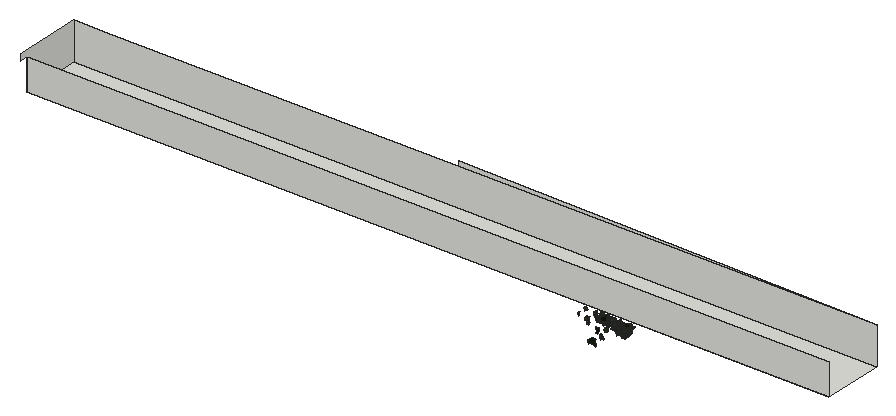
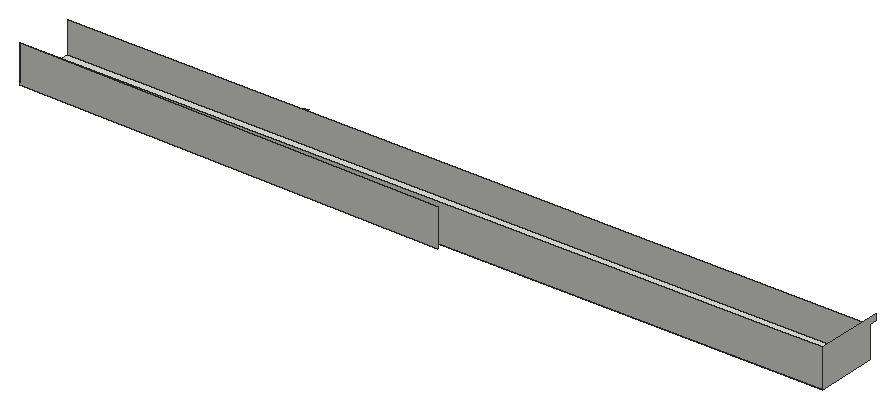
# SketchUp Ruby script. Lengths in inches.
U = 1.inch
M = Sketchup.active_model
def pt(a) = Geom::Point3d.new(a.map { |v| v * U })
def face(e, loops, mat)
  f = e.add_face(loops[0].map { |a| pt(a) })
  loops[1..].each { |l| e.add_face(l.map { |a| pt(a) }).erase! }
  f.material = f.back_material = mat if mat
  f
end
# faces: each face lists its corners as indices into pts; further lists are holes
def faces(e, pts, list, mat = nil) = list.each { |f| face(e, (f[0].is_a?(Array) ? f : [f]).map { |l| l.map { |i| pts[i] } }, mat) }
# xy, xz, yz: faces in a plane at the given z, y or x. An outline is a flat list of corners, or four numbers for a rectangle; further outlines are holes
def ring(l) = l.size == 4 ? [[l[0], l[1]], [l[2], l[1]], [l[2], l[3]], [l[0], l[3]]] : l.each_slice(2).to_a
def flat(e, list, mat, &to3) = list.each { |f| face(e, (f[0].is_a?(Array) ? f : [f]).map { |l| ring(l).map { |u, v| to3.(u, v) } }, mat) }
def xy(e, z, list, mat = nil) = flat(e, list, mat) { |x, y| [x, y, z] }
def xz(e, y, list, mat = nil) = flat(e, list, mat) { |x, z| [x, y, z] }
def yz(e, x, list, mat = nil) = flat(e, list, mat) { |y, z| [x, y, z] }
def lines(e, pts, list) = list.each { |a, b| e.add_line(pt(pts[a]), pt(pts[b])) }
# prism: a flat outline (further loops are holes) pulled along v
def prism(e, loops, v, mat = nil)
  f = face(e, loops, mat); d = Geom::Vector3d.new(v.map { |x| x * U })
  f.pushpull(f.normal.samedirection?(d) ? d.length : -d.length)
end
def box(e, o, s, mat = nil) = prism(e, [[o, [o[0] + s[0], o[1], o[2]], [o[0] + s[0], o[1] + s[1], o[2]], [o[0], o[1] + s[1], o[2]]]], [0, 0, s[2]], mat)
def at(x, y, z, deg = 0) = Geom::Transformation.translation(pt([x, y, z])) * Geom::Transformation.rotation(ORIGIN, Z_AXIS, deg.degrees)
def axes(o, x, y, z) = Geom::Transformation.new([*x, 0, *y, 0, *z, 0, *pt(o).to_a, 1])
def part(name) = M.definitions.add(name)
# library, detail: a bought-in or finely detailed component or shape, given as its bounding box
def library(name, o, s) = part(name).tap { |d| box(d.entities, o, s) }
def detail(e, o, s) = box(e.add_group.entities, o, s)
def put(e, d, t, mat = nil) = e.add_instance(d, t).tap { |i| i.material = mat if mat }
def group(e, t, mat = nil) = e.add_group.tap { |g| g.transformation = t; g.material = mat if mat }.entities
root = M.entities
M.materials.add("efeu1").color = [18, 25, 13]
M.materials.add("efeu2").color = [43, 57, 29]
c1 = part("ivyleaf_10")
p = [[0,0.5,-0.03],[-0.0625,2.02,-0.43],[-0.19,2.01,-0.46],[-0.54,1.05,-0.29],[-0.52,0.625,-0.18],[-0.83,0.76,-0.28],
  [-1.16,0.64,-0.33],[-1.15,0.33,-0.24],[-0.77,-0.39,0.02],[-0.3,-0.51,0.16],[0.04,-0.48,0.23],[-0.02,2.01,-0.4375],
  [-0.06,2.01,-0.43],[0.04,-0.49,0.23],[0.67,-0.49,0.14],[1.38,0.36,-0.2],[1.375,0.51,-0.24],[0.81,0.65,-0.19],
  [0.62,0.59,-0.15],[0.6,1.09,-0.28],[0.5,1.23,-0.31]]
faces(c1.entities,p,[[0,1,2,3,4,5,6,7,8,9,10],[11,12,0,13,14,15,16,17,18,19,20]],"efeu2")
c2 = part("ivyleaf_9")
p = [[1.54,2.16,1.25],[1.36,2.04,1.19],[-0.21,0.99,0.68],[-0.71,1.11,0.82],[-0.85,0.86,0.67],[-0.8,0.17,0.21],
  [-0.9,-0.01,0.1],[-0.67,-0.16,-0.02],[-0.08,-0.08,-0.05],[-0.03,-0.6,-0.4],[0.65,-0.88,-0.66],[0.83,-0.6,-0.49],
  [1.29,-0.42,-0.43],[1.8125,-0.07,-0.26],[1.21,0.44,0.15]]
faces(c2.entities,p,[[0,1,2,3,4,5,6,7,8,9,10,11,12,13,14]],"efeu1")
xy(root,154.12,[[244.11,139.97,243.67,166.9375,600,172.6875,600.44,145.72]])
xz(root,172.6875,[[412.26,154.12,600,171.1]])
p = [[243.67,166.9375,171.1],[243.67,166.9375,154.12],[244.11,139.97,154.12],[244.11,139.97,168.16],[244.16,136.53,168.16],[244.16,136.53,171.1],
  [600.44,145.72,154.12],[600.44,145.72,168.16],[260.85,167.21,171.1],[600,172.6875,171.1],[600,172.6875,154.12]]
faces(root,p,[[0,1,2,3,4,5],[6,7,3,2],[8,9,10,1,0]])
put(root,c1,axes([494.1875,137.87,154.14],[0.47272,-0.38948,0.22707],[0.17708,-0.14216,-0.6125],[0.41461,0.50479,0.0027]))
put(root,c1,axes([496.87,138.41,156.75],[0.62684,-0.04431,-0.10252],[-0.10228,0.00702,-0.6284],[0.04486,0.63513,-0.0002]))
put(root,c1,axes([499.58,135.4,155.04],[0.33148,0.54304,0.37357],[0.1941,0.31919,-0.63621],[-0.6299,0.38412,0.00054]))
put(root,c1,axes([499.91,135.4,153.21],[0.19119,-0.08958,-0.71251],[0.63493,-0.3234,0.21103],[-0.33551,-0.66305,-0.00667]))
put(root,c1,axes([501.62,137.51,156.94],[-0.27922,-0.41477,-0.49379],[0.27947,0.4071,-0.49998],[0.58117,-0.39503,0.00319]))
put(root,c1,axes([502.09,137.56,154.76],[-0.31674,0.08852,0.62038],[0.60112,-0.15355,0.32881],[0.17712,0.67943,-0.00652]))
put(root,c1,axes([503.05,137.92,153.99],[-0.42973,-0.39488,-0.26374],[0.17751,0.19634,-0.58319],[0.44044,-0.46442,-0.0223]))
put(root,c1,axes([503.26,139.19,156.5],[0.20128,-0.51218,-0.35191],[-0.0623,0.35141,-0.5471],[0.6183,0.20214,0.05944]))
put(root,c1,axes([503.68,138.32,157],[-0.08296,-0.35065,-0.52599],[0.15228,0.50379,-0.35987],[0.61354,-0.17245,0.0182]))
put(root,c1,axes([503.71,138.3,154.38],[-0.2872,0.56478,-0.06141],[0.02675,-0.05529,-0.63361],[-0.56748,-0.28844,0.00121]))
put(root,c1,axes([503.36,136.47,155.96],[-0.12078,0.02245,-0.72965],[0.7174,-0.13318,-0.12285],[-0.13505,-0.72749,-0.00003]))
put(root,c1,axes([503.96,138.3,156.6],[0.02561,-0.2422,-0.61075],[0.13944,0.5993,-0.23181],[0.64206,-0.1205,0.07471]))
put(root,c1,axes([504.64,138.72,153.97],[0.20829,-0.57579,0.19315],[0.0493,-0.18749,-0.61208],[0.60532,0.2134,-0.01661]))
put(root,c1,axes([504.8,138.11,155.21],[0.04315,0.54456,0.35881],[0.03766,0.35691,-0.54621],[-0.65105,0.05674,-0.00781]))
put(root,c1,axes([504.82,138.46,154.46],[0.01472,-0.12796,0.64505],[0.58115,-0.29945,-0.07267],[0.30778,0.57152,0.10635]))
put(root,c1,axes([505.3,138.68,155.97],[0.04591,-0.0821,0.63986],[0.31247,-0.55838,-0.09406],[0.56438,0.31582,0.00003]))
put(root,c1,axes([505.53,138.35,155.77],[-0.03276,-0.53837,-0.3507],[0.10491,0.34196,-0.53476],[0.6339,-0.08442,0.07038]))
put(root,c1,axes([505.6875,137.77,153.86],[0.12879,-0.42891,-0.45533],[0.03179,0.46877,-0.43258],[0.62472,0.06457,0.11588]))
put(root,c1,axes([505.8,136.53,154.77],[-0.50095,-0.5107,0.08638],[0.06584,0.05641,0.71534],[-0.51375,0.50521,0.00744]))
put(root,c1,axes([506.09,139.25,156.3],[0.36935,-0.56109,0.06381],[0.03359,-0.05428,-0.67174],[0.56371,0.37087,-0.00178]))
put(root,c1,axes([505.95,136.48,154.76],[-0.1966,0.05078,0.69356],[0.66825,-0.18571,0.20302],[0.19249,0.69656,0.00356]))
put(root,c2,axes([506.57,135.91,156.34],[-0.10299,-0.125,0.77139],[0.6412,0.43123,0.15549],[-0.44668,0.64784,0.04534]))
put(root,c2,axes([507.37,132,153.63],[-0.11051,0.25647,0.79575],[-0.34347,0.69603,-0.28687],[-0.80101,-0.33385,0.01322]))
put(root,c1,axes([506.59,138.27,153.61],[-0.06504,-0.25527,-0.60484],[0.47045,0.4058,-0.22186],[0.45789,-0.45319,0.14203]))
put(root,c1,axes([506.49,137.82,154.75],[-0.28431,0.07812,-0.60434],[0.58786,-0.14041,-0.29471],[-0.16043,-0.65294,-0.00893]))
put(root,c1,axes([507.09,137.67,155.21],[-0.62974,-0.1172,-0.22907],[0.22439,0.04626,-0.64054],[0.12593,-0.66851,-0.00417]))
put(root,c1,axes([507.59,138.34,154.75],[0.59498,0.02493,0.31027],[-0.31001,-0.01268,0.5955],[0.02797,-0.6709,0.00028]))
put(root,c1,axes([507.58,139.08,155.28],[0.00841,-0.63597,0.24737],[0.00964,-0.24725,-0.636],[0.68231,0.01134,0.00594]))
put(root,c1,axes([507.3,139.05,153.1875],[0.12422,0.04086,-0.62839],[0.61765,0.11687,0.1297],[0.12268,-0.6298,-0.0167]))
put(root,c1,axes([508.14,138,155.15],[0.2574,-0.27645,-0.58411],[-0.38255,0.44155,-0.37756],[0.52083,0.46095,0.01136]))
put(root,c1,axes([507.82,135.92,155.61],[-0.33657,-0.4779,-0.51375],[0.27841,0.43207,-0.58431],[0.64407,-0.43651,-0.01589]))
put(root,c1,axes([508.07,138.49,155.84],[-0.04785,-0.32684,0.54806],[0.06779,-0.54909,-0.32154],[0.63451,0.03402,0.07568]))
put(root,c1,axes([507.66,138.15,156.55],[-0.0112,-0.09365,0.63728],[0.62192,-0.16748,-0.01369],[0.16766,0.61498,0.09332]))
put(root,c1,axes([508.18,137.2,156.92],[0.40119,-0.42822,0.30697],[0.19968,-0.23347,-0.58667],[0.48757,0.44797,-0.01232]))
put(root,c1,axes([507.93,138.93,155.86],[-0.1383,-0.088,0.63625],[0.5033,0.3895,0.16327],[-0.39905,0.52176,-0.01458]))
put(root,c1,axes([508.59,137.17,156.5625],[-0.10409,-0.57947,0.32447],[0.00212,-0.32872,-0.58638],[0.66412,-0.08977,0.05272]))
put(root,c1,axes([508.49,135,153.72],[0.28079,0.5323,0.37246],[0.14121,0.33435,-0.61555],[-0.67834,0.28994,0.02604]))
put(root,c1,axes([508.46,138.41,155.38],[-0.03751,-0.12566,-0.6279],[0.50713,0.37821,-0.10598],[0.39099,-0.50261,0.07723]))
put(root,c1,axes([509.22,136.29,155.34],[-0.1846,0.20082,-0.59137],[-0.4276,0.40844,0.27379],[0.49126,0.43096,0.01609]))
put(root,c1,axes([508.68,138.54,153.67],[-0.2405,-0.26948,-0.52768],[0.36173,0.38427,-0.36111],[0.46928,-0.43431,0.00791]))
put(root,c1,axes([508.7,138.22,154.71],[0.2227,0.48137,0.36426],[0.15461,0.32983,-0.53038],[-0.58352,0.2711,-0.00151]))
put(root,c1,axes([509.35,136.75,154.99],[0.31739,-0.03122,0.5504],[-0.56995,0.04049,0.30726],[-0.05461,-0.604,-0.00786]))
put(root,c1,axes([509.45,138.48,153.24],[-0.02222,-0.47314,-0.47227],[0.09474,0.46553,-0.47084],[0.66175,-0.08253,0.05155]))
put(root,c1,axes([509.37,138.04,153.14],[-0.61391,-0.21507,-0.27299],[0.25668,0.09296,-0.65049],[0.23429,-0.66541,-0.00264]))
put(root,c1,axes([509.27,137.54,156.08],[0.22465,0.16439,-0.57322],[0.44832,0.35734,0.27818],[0.3932,-0.50135,0.01032]))
put(root,c1,axes([509.83,137.66,153.75],[-0.0912,0.49591,0.41119],[-0.06996,0.40521,-0.50421],[-0.6404,-0.11489,-0.00348]))
put(root,c1,axes([509.9375,138.02,153.875],[0.08417,-0.32764,-0.55839],[0.02804,0.5644,-0.32694],[0.64681,0.01817,0.08684]))
put(root,c1,axes([510.47,138.07,156.65],[0.05983,-0.04414,-0.63331],[-0.32343,0.54526,-0.06856],[0.54628,0.32766,0.02877]))
put(root,c1,axes([510.2,137.79,155.61],[0.07077,-0.20673,0.62952],[0.23537,-0.58396,-0.21823],[0.61938,0.24553,0.011]))
put(root,c1,axes([510.18,138.52,156.22],[-0.46721,0.39163,-0.24482],[0.19247,-0.15147,-0.6096],[-0.41984,-0.50525,-0.00702]))
put(root,c2,axes([510.08,124.95,154.44],[-0.04384,-0.59722,-0.80018],[0.11698,0.76253,-0.6215],[1.04538,-0.11037,0.03599]))
put(root,c1,axes([510.41,137.89,155.25],[-0.65668,-0.2154,0.2012],[0.19337,0.05598,0.69107],[-0.22246,0.68452,0.0068]))
put(root,c1,axes([510.46,137.83,154.05],[0.08125,-0.00523,-0.64762],[0.62994,-0.15092,0.08025],[-0.15038,-0.63501,-0.01374]))
put(root,c1,axes([511.58,138.12,155.14],[0.02506,0.02157,0.63713],[-0.53268,-0.34957,0.03279],[0.35021,-0.53325,0.00428]))
put(root,c1,axes([510.57,129.66,153.82],[0.10998,-0.05164,0.86236],[0.88971,-0.10192,-0.11182],[0.11621,0.82918,0.03996]))
put(root,c1,axes([511.25,138,152.68],[-0.59375,-0.18347,0.21102],[0.20712,0.0442,0.62119],[-0.18786,0.62858,0.01791]))
put(root,c1,axes([511.88,137.58,154.3],[0.45564,0.14801,-0.46596],[-0.44319,-0.14387,-0.47908],[-0.20641,0.63563,0.00007]))
put(root,c1,axes([511.23,136.9,155.18],[0.36826,0.10938,-0.51488],[0.49425,0.14429,0.38416],[0.18106,-0.61636,-0.00144]))
put(root,c1,axes([511.92,138.5,155.11],[-0.00412,-0.64851,-0.13381],[-0.00769,0.13385,-0.64847],[0.66213,-0.00248,-0.00837]))
put(root,c1,axes([511.6875,139.77,154.3],[-0.32096,-0.43006,0.38361],[0.23195,0.30555,0.53663],[-0.52755,0.396,0.00255]))
put(root,c1,axes([512.33,138.04,154.96],[-0.1427,0.28396,-0.56339],[-0.31996,0.46526,0.31554],[0.54376,0.34829,0.03782]))
put(root,c1,axes([511.89,138.14,154.29],[0.37754,0.4355,-0.28324],[0.18797,0.21189,0.57636],[0.48431,-0.42173,-0.00291]))
put(root,c1,axes([511.9375,137.08,154.03],[0.34678,-0.51478,0.30275],[0.15979,-0.25734,-0.62061],[0.57543,0.38169,-0.01011]))
put(root,c1,axes([512.27,138.69,156.375],[0.44796,-0.40554,-0.30883],[-0.23029,0.20578,-0.60426],[0.45476,0.50369,-0.00178]))
put(root,c1,axes([512.375,138.23,153.58],[0.54721,-0.3876,0.19874],[-0.15518,0.12469,0.67047],[-0.407,-0.56867,0.01156]))
put(root,c1,axes([512.38,137.67,156.66],[-0.07455,0.65091,-0.32371],[0.03033,-0.32234,-0.65514],[-0.72633,-0.08027,0.00587]))
put(root,c1,axes([512.25,136.7,155.06],[0.21999,0.06257,-0.60972],[0.49227,0.36791,0.21537],[0.36517,-0.53367,0.07699]))
put(root,c1,axes([512.61,136.64,156.49],[0.25246,-0.61681,0.30711],[0.16377,-0.26399,-0.66483],[0.66929,0.29726,0.04683]))
put(root,c1,axes([512.6,137.14,153.15],[-0.01837,0.05324,0.71324],[0.23801,-0.67236,0.05632],[0.67446,0.23872,-0.00045]))
put(root,c1,axes([512.48,136.71,156.34],[0.33058,-0.40707,0.46381],[0.34055,-0.31845,-0.52222],[0.51463,0.47221,0.04764]))
put(root,c1,axes([512.57,137.47,154.66],[0.36503,0.54256,0.17209],[0.08927,0.14733,-0.65387],[-0.56215,0.3757,0.0079]))
put(root,c1,axes([512.73,137.4,155.83],[-0.11597,-0.56844,0.34966],[0.06809,0.34297,0.58014],[-0.66389,0.13447,-0.00158]))
put(root,c1,axes([513.29,136.96,153.16],[-0.08183,-0.34307,0.6304],[-0.01076,-0.63382,-0.34633],[0.71762,-0.04862,0.06669]))
put(root,c1,axes([513.44,136.49,153.65],[-0.39422,-0.632,0.01407],[-0.00448,-0.0138,-0.74486],[0.63214,-0.39423,0.0035]))
put(root,c1,axes([513.39,137.46,155.45],[-0.39088,-0.5114,-0.17382],[-0.10859,-0.13577,0.64367],[-0.52911,0.40566,-0.0037]))
put(root,c1,axes([513.55,138.57,155.14],[0.07985,-0.01841,-0.68233],[-0.17978,0.66217,-0.03891],[0.65848,0.18301,0.07212]))
put(root,c1,axes([513.62,138.58,154.04],[0.1807,-0.66787,0.01791],[0.0047,-0.01728,-0.69189],[0.6681,0.18077,0.00002]))
put(root,c1,axes([513.69,136.92,157.07],[0.0103,-0.59538,0.43075],[0.06383,-0.42844,-0.59371],[0.73209,0.04573,0.04571]))
put(root,c1,axes([513.83,138.12,154.87],[-0.54916,-0.37019,0.07828],[-0.06504,-0.04356,-0.66228],[0.37274,-0.553,-0.00024]))
put(root,c1,axes([513.35,137.9,156.41],[-0.2657,-0.03052,0.58921],[0.58322,0.08414,0.26735],[-0.08922,0.64085,-0.00704]))
put(root,c1,axes([513.35,136.67,156.45],[-0.04916,-0.06909,0.70286],[0.64485,0.28293,0.07291],[-0.28801,0.64527,0.04328]))
put(root,c1,axes([513.6,137.3125,154.6],[-0.02661,0.0114,0.75508],[0.74086,0.14678,0.02389],[-0.14631,0.74116,-0.01635]))
put(root,c1,axes([514.18,138.78,154.27],[0.4898,-0.42809,0.11067],[0.08415,-0.07188,-0.65051],[0.43408,0.49698,0.00124]))
put(root,c2,axes([514.12,136.73,154.47],[-0.39197,-0.20725,-0.62022],[0.53956,0.30604,-0.44326],[0.36946,-0.66683,-0.01067]))
put(root,c1,axes([514.61,139.21,155],[0.09402,-0.17676,0.63852],[-0.26721,0.58002,0.19991],[-0.60626,-0.28306,0.01091]))
put(root,c1,axes([514.875,137.68,155.46],[0.02848,0.09722,0.66532],[-0.3725,-0.55211,0.09662],[0.55977,-0.37234,0.03044]))
put(root,c1,axes([514.55,136.66,153.5],[-0.30154,-0.58911,-0.31887],[0.17894,0.26614,-0.66091],[0.64553,-0.34896,0.03425]))
put(root,c1,axes([514.61,136.75,153.84],[-0.14876,-0.39023,-0.5446],[0.24552,0.4873,-0.41624],[0.62337,-0.28506,0.03398]))
put(root,c1,axes([515.1,138.3,154.58],[-0.22417,-0.25606,0.61545],[-0.30984,-0.53489,-0.3354],[0.59021,-0.37805,0.05768]))
put(root,c1,axes([514.75,137.98,152.85],[-0.07553,-0.60993,0.28193],[0.03641,0.27957,0.61458],[-0.67095,0.08383,0.00162]))
put(root,c1,axes([514.6,136.92,153.36],[-0.19502,-0.19922,-0.6954],[0.50063,0.48271,-0.27869],[0.52215,-0.53722,0.00747]))
put(root,c1,axes([514.6,136.43,152.55],[0.3992,0.02486,-0.58698],[0.52863,0.29446,0.37199],[0.25636,-0.64591,0.14699]))
put(root,c1,axes([514.57,136.8,153.41],[-0.15599,0.01189,0.72121],[0.70717,-0.14288,0.15531],[0.14214,0.72392,0.01881]))
put(root,c1,axes([514.6,136.39,156.18],[0.07738,0.00514,0.66847],[0.64856,0.16251,-0.07633],[-0.16201,0.65301,0.01374]))
put(root,c1,axes([515.35,137.12,155.51],[0.18752,-0.34002,-0.50703],[-0.24688,0.44287,-0.3883],[0.55834,0.31002,-0.0014]))
put(root,c1,axes([515.19,136.97,156.375],[-0.34171,-0.53042,-0.18311],[0.10572,0.14969,-0.63092],[0.55109,-0.35761,0.00749]))
put(root,c1,axes([515.2,136.4,153.125],[-0.5584,-0.41819,-0.1508],[0.12304,0.08727,-0.69762],[0.42718,-0.57178,0.00381]))
put(root,c1,axes([515.7,136.26,156.73],[0.19107,-0.15762,-0.59616],[-0.44749,0.39397,-0.24758],[0.42427,0.48652,0.00734]))
put(root,c1,axes([515.44,137.24,154.49],[0.24651,-0.61543,-0.20288],[-0.07753,0.18749,-0.66296],[0.64335,0.25841,-0.00216]))
put(root,c1,axes([515.63,136.8,154.72],[0.22707,0.3104,-0.62414],[-0.39543,-0.48321,-0.38418],[-0.57404,0.45564,0.01776]))
put(root,c1,axes([515.36,136.3125,155.11],[-0.15954,-0.07535,-0.64788],[0.60751,0.2256,-0.17583],[0.23741,-0.62794,0.01457]))
put(root,c1,axes([515.59,136.26,155.25],[0.55235,0.28289,0.14096],[0.12049,0.07392,-0.62049],[-0.2922,0.56524,0.0106]))
put(root,c1,axes([515.94,138.21,154.67],[0.42205,0.40958,0.25548],[-0.18257,-0.17872,0.58812],[0.44688,-0.45985,-0.00102]))
put(root,c1,axes([515.99,137.53,153.33],[0.28248,-0.63719,0.02041],[0.00802,-0.01877,-0.69699],[0.63746,0.28259,-0.00027]))
put(root,c1,axes([515.91,138.26,152.25],[0.61199,-0.24836,0.05896],[-0.04453,0.04695,0.65992],[-0.25135,-0.61303,0.02665]))
put(root,c1,axes([515.86,137.79,153.79],[-0.21211,-0.39566,0.52059],[0.24243,0.46071,0.44892],[-0.60728,0.32211,-0.00262]))
put(root,c1,axes([515.62,136.36,152.84],[-0.04489,-0.04702,0.64051],[0.64098,-0.04341,0.04173],[0.04014,0.64061,0.04984]))
put(root,c1,axes([515.83,137.34,155.95],[0.54624,-0.29907,-0.35737],[0.32491,-0.15029,0.62239],[-0.33405,-0.63521,0.02099]))
put(root,c1,axes([516.66,138.68,153.78],[0.43215,-0.30044,-0.52789],[-0.42956,0.30687,-0.52631],[0.42943,0.60931,0.00478]))
put(root,c1,axes([516.7,135.92,155.17],[-0.14027,-0.21471,0.59454],[-0.28136,-0.52415,-0.25567],[0.56605,-0.31374,0.02025]))
put(root,c1,axes([516.52,139.21,156.18],[0.6468,-0.0717,-0.12679],[-0.12571,0.01675,-0.65076],[0.07358,0.6589,0.00275]))
put(root,c1,axes([516.9375,138.6875,153.85],[0.34548,-0.25995,-0.6108],[-0.47275,0.38703,-0.43212],[0.46601,0.58536,0.01446]))
put(root,c1,axes([516.25,136.36,155.62],[0.46879,0.29374,-0.55906],[0.48684,0.27541,0.55294],[0.40227,-0.67562,-0.01767]))
put(root,c1,axes([516.64,137.27,153.53],[0.34266,-0.53548,0.23816],[0.12502,-0.20274,-0.63572],[0.57256,0.36474,-0.00371]))
put(root,c1,axes([517.04,137.26,154.8],[0.15836,0.2977,0.55175],[-0.24597,-0.49395,0.33711],[0.57667,-0.29244,-0.00773]))
put(root,c1,axes([516.9,137.87,156.05],[0.12508,-0.64797,-0.11141],[-0.02717,0.10822,-0.65991],[0.65692,0.12786,-0.00608]))
put(root,c1,axes([516.85,136.62,153.49],[0.25327,-0.63964,0.08936],[0.02822,-0.08493,-0.68794],[0.64524,0.25479,-0.00498]))
put(root,c2,axes([516.77,136.74,157.375],[-0.49291,-0.46271,-0.41312],[0.29778,0.28638,-0.67605],[0.54415,-0.57586,-0.00426]))
put(root,c1,axes([517.14,136.16,156.25],[-0.61793,-0.44909,0.02119],[-0.01235,-0.01904,-0.76384],[0.44942,-0.618,0.00814]))
put(root,c1,axes([516.84,138.69,155.28],[-0.01183,-0.06652,0.67021],[0.14332,0.65471,0.06751],[-0.65808,0.14378,0.00266]))
